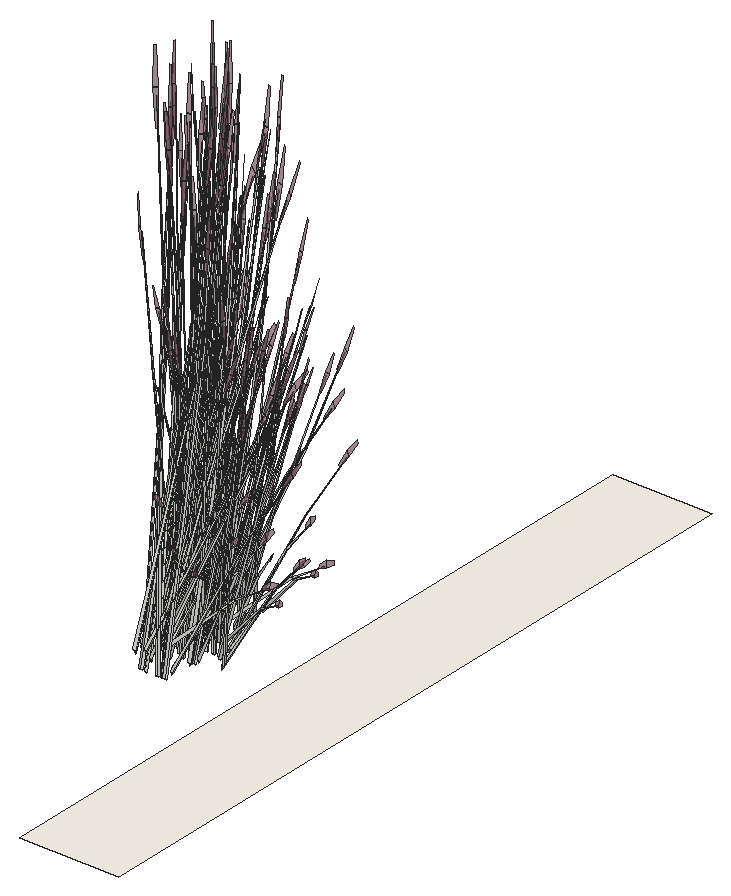
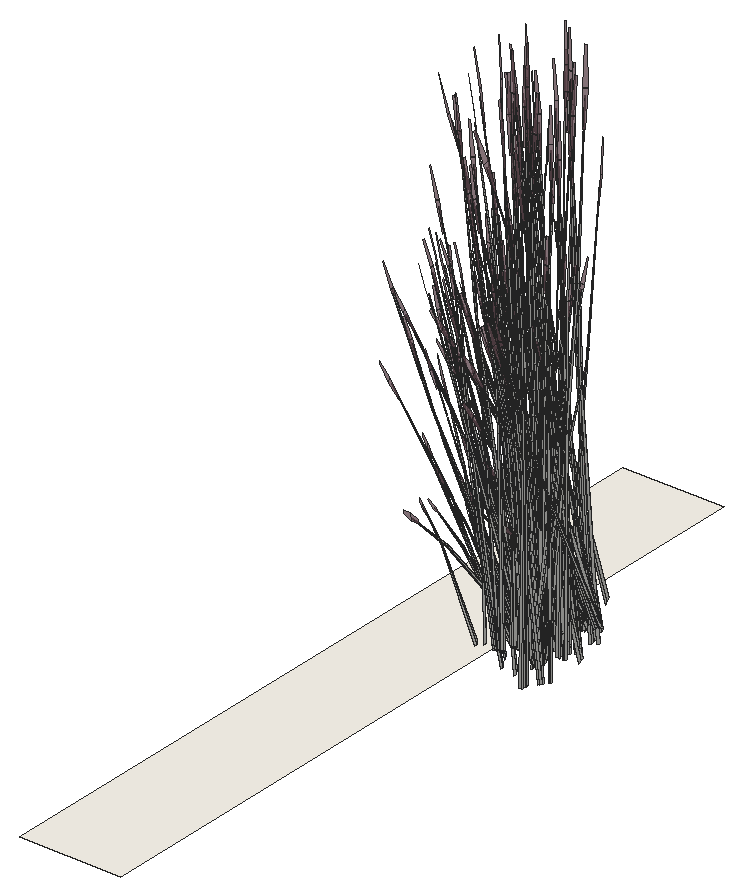
# SketchUp Ruby script. Lengths in inches.
U = 1.inch
M = Sketchup.active_model
def pt(a) = Geom::Point3d.new(a.map { |v| v * U })
def face(e, loops, mat)
  f = e.add_face(loops[0].map { |a| pt(a) })
  loops[1..].each { |l| e.add_face(l.map { |a| pt(a) }).erase! }
  f.material = f.back_material = mat if mat
  f
end
# faces: each face lists its corners as indices into pts; further lists are holes
def faces(e, pts, list, mat = nil) = list.each { |f| face(e, (f[0].is_a?(Array) ? f : [f]).map { |l| l.map { |i| pts[i] } }, mat) }
# xy, xz, yz: faces in a plane at the given z, y or x. An outline is a flat list of corners, or four numbers for a rectangle; further outlines are holes
def ring(l) = l.size == 4 ? [[l[0], l[1]], [l[2], l[1]], [l[2], l[3]], [l[0], l[3]]] : l.each_slice(2).to_a
def flat(e, list, mat, &to3) = list.each { |f| face(e, (f[0].is_a?(Array) ? f : [f]).map { |l| ring(l).map { |u, v| to3.(u, v) } }, mat) }
def xy(e, z, list, mat = nil) = flat(e, list, mat) { |x, y| [x, y, z] }
def xz(e, y, list, mat = nil) = flat(e, list, mat) { |x, z| [x, y, z] }
def yz(e, x, list, mat = nil) = flat(e, list, mat) { |y, z| [x, y, z] }
def lines(e, pts, list) = list.each { |a, b| e.add_line(pt(pts[a]), pt(pts[b])) }
# prism: a flat outline (further loops are holes) pulled along v
def prism(e, loops, v, mat = nil)
  f = face(e, loops, mat); d = Geom::Vector3d.new(v.map { |x| x * U })
  f.pushpull(f.normal.samedirection?(d) ? d.length : -d.length)
end
def box(e, o, s, mat = nil) = prism(e, [[o, [o[0] + s[0], o[1], o[2]], [o[0] + s[0], o[1] + s[1], o[2]], [o[0], o[1] + s[1], o[2]]]], [0, 0, s[2]], mat)
def at(x, y, z, deg = 0) = Geom::Transformation.translation(pt([x, y, z])) * Geom::Transformation.rotation(ORIGIN, Z_AXIS, deg.degrees)
def axes(o, x, y, z) = Geom::Transformation.new([*x, 0, *y, 0, *z, 0, *pt(o).to_a, 1])
def part(name) = M.definitions.add(name)
# library, detail: a bought-in or finely detailed component or shape, given as its bounding box
def library(name, o, s) = part(name).tap { |d| box(d.entities, o, s) }
def detail(e, o, s) = box(e.add_group.entities, o, s)
def put(e, d, t, mat = nil) = e.add_instance(d, t).tap { |i| i.material = mat if mat }
def group(e, t, mat = nil) = e.add_group.tap { |g| g.transformation = t; g.material = mat if mat }.entities
root = M.entities
M.materials.add("C01_Vanilla_Cream").color = [255, 251, 241]
M.materials.add("LightPink_Translucent").color = [144, 107, 117]
M.materials["LightPink_Translucent"].alpha = 0.75
c1 = part("blade")
p = [[2.15,0.21,22],[0,0.17,0],[0.09,0.45,0],[2.18,0.31,22],[2.29,0.31,22],[0.38,0.45,0],
  [2.48,0.24,33],[2.49,0.24,33],[2.48,0.22,33]]
faces(c1.entities,p,[[0,1,2,3],[4,5,2,3],[6,3,4,7],[8,0,3,6]])
c2 = part("seeds")
p = [[0.3,-0.1,1.38],[-0.01,-0.03,1.59],[-0.01,-0.03,0.03],[0.14,-0.07,-0.07],[0.29,-0.03,3],[0.15,0.01,3.11]]
faces(c2.entities,p,[[0,1,2,3],[1,0,4,5]],"LightPink_Translucent")
c3 = part("blade with seeds")
put(c3.entities,c1,at(0,0,0))
put(c3.entities,c2,axes([2.4,0.25,30.99],[1.5799,-0.05474,1.17369],[-0.12525,1.92788,0.29478],[-0.07173,-0.02425,1.56792]))
xy(root,390,[[696.41,288,706,360]],"C01_Vanilla_Cream")
put(root,c3,axes([690.39,317.23,392.17],[0.48065,0.34305,0.12018],[-0.40092,0.38703,-0.34318],[-0.1116,0.05232,1.05198]))
put(root,c3,axes([690.22,316.8125,391.91],[-0.60515,-0.49144,-0.05089],[0.60552,-0.49174,0],[-0.02113,-0.01716,1.45724]))
put(root,c3,axes([690.38,316.98,392.26],[0.70648,-0.03525,0.37133],[0.06389,0.58508,-0.17871],[-0.12647,0.0593,1.19224]))
put(root,c3,axes([687.82,313.22,394.19],[0.19614,-0.43908,0.29394],[0.57222,0.12807,-0.37948],[0.05247,0.17678,0.72609]))
put(root,c3,axes([688.87,312.48,391.9],[0.28286,0.65594,-0.0499],[-0.80821,0.22985,0],[0.00988,0.02291,1.42904]))
put(root,c3,axes([689.42,319.33,393.93],[0.47939,-0.19405,0.05337],[0.23464,0.35385,0.42015],[-0.0463,-0.15598,0.64067]))
put(root,c3,axes([690.9,318.29,392.06],[0.60889,-0.28548,0.4121],[0.36394,0.51192,0],[-0.13868,0.06502,1.30728]))
put(root,c3,axes([689,316.25,391.96],[0.28286,0.63846,0.37976],[-0.80821,0.22202,0.14902],[0.00988,-0.11732,1.31851]))
put(root,c3,axes([689.25,319.36,393.93],[0.64106,0.14927,0.39842],[-0.21921,0.49074,0.32852],[-0.03852,-0.19299,0.82444]))
put(root,c3,axes([688.87,316.16,391.83],[0.31565,-0.51449,-0.37133],[0.65588,0.24761,0.17871],[0,-0.1186,1.19224]))
put(root,c3,axes([688.48,321.81,392.02],[0.73304,0.27674,0.19974],[-0.35279,0.57501,0.41502],[0,-0.13255,1.3325]))
put(root,c3,axes([689.68,317.82,391.83],[-0.21227,-0.49226,0],[0.60616,-0.17239,0],[0,0,1.28128]))
put(root,c3,axes([687.9375,313.28,394.13],[0.31051,0.46426,-0.58968],[-0.63919,0.25873,0.07116],[0.07261,0.22432,0.83415]))
put(root,c3,axes([691.21,311.62,391.83],[-0.81312,-0.00457,-0.0413],[0,-0.63814,0.41452],[-0.02555,0.14527,1.31432]))
put(root,c3,axes([688.59,314.78,394.6875],[0.44958,-0.32756,-0.05385],[0.41194,0.35875,-0.24415],[0.029,0.10165,0.8053]))
put(root,c3,axes([687.58,319.72,391.97],[-0.40676,-0.57214,0],[0.68052,-0.31907,-0.42834],[0.15499,-0.07267,1.3588]))
put(root,c3,axes([690.54,316.85,391.83],[-0.31565,0.51449,-0.37133],[-0.65588,-0.24761,0.17871],[0,0.1186,1.19224]))
put(root,c3,axes([689.11,312.7,391.83],[0.65588,0.25634,0],[-0.31565,0.53263,0],[0,0,1.45212]))
put(root,c3,axes([688.17,313.38,393.89],[0.63954,0.14313,-0.42412],[-0.21921,0.49074,-0.32852],[0.05864,0.19758,0.81151]))
put(root,c3,axes([687.625,313.4,394.18],[0.63664,-0.26583,-0.10093],[0.31286,0.47181,-0.56021],[0.084,0.19882,0.85122]))
put(root,c3,axes([691.78,316.54,392.05],[-0.51116,-0.4159,0.14643],[0.51512,-0.4034,0.29122],[-0.05645,0.08494,1.33138]))
put(root,c3,axes([690.02,316.3,391.83],[0,-0.66065,0],[0.81352,0,0],[0,0,1.48949]))
put(root,c3,axes([689.28,318.33,392.3],[0.08346,0.33295,0.95334],[-0.46298,-0.1844,0.70045],[0.04982,-0.17048,0.20998]))
put(root,c3,axes([689.26,316.42,392.02],[0.73304,0.27674,0.19974],[-0.35279,0.57501,0.41502],[0,-0.13255,1.3325]))
put(root,c3,axes([690.43,316.5625,391.9],[0,0.66033,-0.04679],[-0.81352,0,0],[0,0.02075,1.48875]))
put(root,c3,axes([689.03,316.03,392.26],[-0.70648,0.03525,0.37133],[-0.06389,-0.58508,-0.17871],[0.12647,-0.0593,1.19224]))
put(root,c3,axes([691.04,311.72,391.68],[-0.45414,0.35624,-0.25712],[-0.45414,-0.35624,0.25712],[0,0.11474,1.15348]))
put(root,c3,axes([689.74,311.65,391.74],[0.23855,0.52277,-0.57446],[-0.68718,0.18827,-0.15077],[0.02637,0.17702,1.26801]))
put(root,c3,axes([688.7,315.03,392.05],[-0.18794,0.56744,0.14643],[-0.68774,-0.16058,0.29122],[0.1188,-0.00276,1.33138]))
put(root,c3,axes([690.04,317.84,391.9],[0.28286,0.65594,-0.0499],[-0.80821,0.22985,0],[0.00988,0.02291,1.42904]))
put(root,c3,axes([691.26,318.88,393.91],[-0.06607,0.04361,1.47228],[-0.64734,-0.14714,-0.13912],[-0.02343,-0.19032,0.26054]))
put(root,c3,axes([690.75,320.14,394.18],[-0.71502,-0.02829,-0.10093],[0.01954,-0.53563,-0.56021],[0.04967,-0.20629,0.85122]))
put(root,c3,axes([692.375,316.98,391.83],[-0.81312,-0.00457,-0.0413],[0,-0.63814,0.41452],[-0.02555,0.14527,1.31432]))
put(root,c3,axes([689.45,311.07,392.21],[0.73268,0.27244,-0.24149],[-0.35279,0.57501,-0.41502],[0.02303,0.14118,1.32557]))
put(root,c3,axes([690.78,315.0625,392.05],[-0.6991,0.15154,0.14643],[-0.17263,-0.56398,0.29122],[0.06235,0.08217,1.33138]))
put(root,c3,axes([690.47,320.22,394.19],[-0.4402,0.30062,0.29394],[-0.41671,-0.34326,-0.37948],[0.0634,-0.1744,0.72609]))
put(root,c3,axes([688.375,321.3,392.21],[-0.07581,-0.65151,-0.24149],[0.7896,-0.03939,-0.41502],[0.13904,-0.08678,1.32557]))
put(root,c3,axes([690.27,319.93,393.89],[-0.46573,-0.38364,-0.42412],[0.49199,-0.33598,-0.32852],[0.07086,-0.19492,0.81151]))
put(root,c3,axes([689.63,315.88,391.96],[-0.53943,0.51816,0.37976],[-0.64086,-0.4574,0.14902],[0.13005,-0.05171,1.31851]))
put(root,c3,axes([690.55,316.7,391.84],[0.45414,0.3688,0],[-0.45414,0.3688,0],[0,0,1.40491]))
put(root,c3,axes([690.55,316.27,392.26],[0.31565,-0.51449,0.37133],[0.65588,0.24761,-0.17871],[0,0.1186,1.19224]))
put(root,c3,axes([690.27,318.06,391.83],[0.65588,0.25634,0],[-0.31565,0.53263,0],[0,0,1.45212]))
put(root,c3,axes([691.35,311.73,391.67],[0,0.57097,-0.4121],[-0.72788,0,0],[0,0.13004,1.30728]))
put(root,c3,axes([689.4,313.46,393.93],[-0.64708,0.13103,0.39842],[-0.1123,-0.514,0.32852],[0.15218,0.15149,0.82444]))
put(root,c3,axes([689.28,313.56,393.93],[-0.29569,0.36271,0.05337],[-0.42107,-0.21117,0.42015],[0.13613,0.11629,0.64067]))
put(root,c3,axes([688.53,312.36,393.22],[-0.14872,-0.18332,1.42242],[0.6872,-0.15433,0.11501],[0.15531,0.28779,0.60807]))
put(root,c3,axes([688.27,319.85,391.68],[0.60696,0.14127,-0.25712],[-0.15283,0.49751,0.25712],[0.12236,-0.05737,1.15348]))
put(root,c3,axes([690.34,316.15,391.98],[-0.82229,-0.1203,0.40835],[0.16734,-0.67942,0.16024],[0.12017,0.06561,1.41775]))
put(root,c3,axes([689.96,319.25,392.15],[-0.18493,0.11557,1.18691],[-0.55384,-0.20228,-0.25526],[0.10266,-0.25157,0.50747]))
put(root,c3,axes([692.21,317.07,391.68],[-0.45414,0.35624,-0.25712],[-0.45414,-0.35624,0.25712],[0,0.11474,1.15348]))
put(root,c3,axes([688.13,319.63,391.67],[0.60889,-0.28548,-0.4121],[0.36394,0.51192,0],[0.13868,-0.06502,1.30728]))
put(root,c3,axes([690.57,316.45,391.83],[0.72788,0,0],[0,0.59111,0],[0,0,1.48078]))
put(root,c3,axes([689.87,315.8,392.26],[-0.39083,-0.47924,0.37133],[0.59199,-0.33747,-0.17871],[0.12647,0.0593,1.19224]))
put(root,c3,axes([689.16,315.91,392.21],[-0.07581,-0.65151,-0.24149],[0.7896,-0.03939,-0.41502],[0.13904,-0.08678,1.32557]))
put(root,c3,axes([690.82,316.39,392.17],[0.60616,-0.16651,0.12018],[0.21227,0.47548,-0.34318],[0,0.10465,1.05198]))
put(root,c3,axes([690.41,320.11,394.13],[0.01693,-0.52814,-0.58968],[0.71285,0.03547,0.07116],[0.07523,-0.22375,0.83415]))
put(root,c3,axes([689.1875,313.14,394.19],[-0.10048,-0.4599,0.29394],[0.5744,-0.12144,-0.37948],[0.15428,0.13179,0.72609]))
put(root,c3,axes([690.62,316.43,392.21],[0.73268,0.27244,-0.24149],[-0.35279,0.57501,-0.41502],[0.02303,0.14118,1.32557]))
put(root,c3,axes([689.06,314.47,391.68],[0.60696,0.14127,-0.25712],[-0.15283,0.49751,0.25712],[0.12236,-0.05737,1.15348]))
put(root,c3,axes([689.58,310.5,393.71],[-0.56218,-0.29666,1.14775],[0.59361,-0.46189,0.49522],[0.18138,0.27836,1.10941]))
put(root,c3,axes([688.63,313.79,393.91],[0.00193,-0.06913,1.47228],[0.55753,-0.30498,-0.13912],[0.19366,0.10886,0.26054]))
put(root,c3,axes([690.42,312.91,392.3],[-0.36631,-0.16417,0.95334],[0.47299,-0.16681,0.70045],[0.12758,0.1413,0.20998]))
put(root,c3,axes([689.12,312.74,392.15],[0.01148,-0.18927,1.18691],[0.54864,-0.21141,-0.25526],[0.16937,0.22654,0.50747]))
put(root,c3,axes([692.21,316.56,392.06],[0,-0.57097,0.4121],[0.72788,0,0],[0,0.13004,1.30728]))
put(root,c3,axes([690.13,315.66,392.17],[0.12551,-0.50956,0.12018],[0.6132,0.08845,-0.34318],[0.1116,0.05232,1.05198]))
put(root,c3,axes([690.7,319.79,393.76],[0.4402,-0.30062,-0.29394],[0.41671,0.34326,0.37948],[0.0634,-0.1744,0.72609]))
put(root,c3,axes([690.87,319.95,393.93],[0.53464,0.0266,0.05337],[-0.01466,0.40172,0.42015],[0.05594,-0.15388,0.64067]))
put(root,c3,axes([691.53,311.29,391.97],[0.81352,0,0],[0,0.63814,-0.42834],[0,0.14534,1.3588]))
put(root,c3,axes([691.01,314.77,392.06],[-0.60889,-0.28548,0.4121],[0.36394,-0.51192,0],[0.13868,0.06502,1.30728]))
put(root,c3,axes([691.4,319.29,393.91],[-0.00628,-0.11364,1.45204],[-0.53042,-0.32843,-0.22964],[0.08201,-0.19909,0.11645]))
put(root,c3,axes([688.85,320.8,391.71],[0.43821,-0.42916,-0.51753],[0.54436,0.38915,-0.13583],[0.1756,-0.10706,1.14236]))
put(root,c3,axes([690.7,319.91,393.93],[0.46327,0.38957,0.39842],[-0.49199,0.33598,0.32852],[0.08546,-0.18277,0.82444]))
put(root,c3,axes([690.47,317.75,391.8125],[0.68303,-0.19373,-0.15934],[0.24001,0.55805,0.00007],[0.07539,-0.02141,1.44335]))
put(root,c3,axes([690.48,313.66,392.21],[-0.4172,-0.01791,0.872],[0.27552,-0.38032,0.48145],[0.16481,0.13512,0.68401]))
put(root,c3,axes([690.49,316.1,391.83],[0.39083,0.47924,-0.37133],[-0.59199,0.33747,0.17871],[0.12647,0.0593,1.19224]))
put(root,c3,axes([691.24,321.15,394.19],[-0.56631,0.0816,0.29394],[-0.14954,-0.46647,-0.37948],[0.16229,-0.12529,0.72609]))
put(root,c3,axes([689.14,313.38,394.18],[0.38768,-0.48872,-0.10093],[0.56143,0.28156,-0.56021],[0.19516,0.13808,0.85122]))
put(root,c3,axes([689.61,319.84,393.22],[-0.12114,0.19625,1.42242],[-0.50818,-0.40613,0.11501],[0.22925,-0.25313,0.60807]))
put(root,c3,axes([689.63,315.41,391.71],[0.43821,-0.42916,-0.51753],[0.54436,0.38915,-0.13583],[0.1756,-0.10706,1.14236]))
put(root,c3,axes([689.6,313.14,393.89],[0.64198,-0.13573,-0.42412],[0.1123,0.514,-0.32852],[0.17243,0.1473,0.81151]))
put(root,c3,axes([690.33,312.52,394.19],[-0.37017,-0.35748,0.29394],[0.42268,-0.3384,-0.37948],[0.21476,0.05149,0.72609]))
put(root,c3,axes([691.53,321.19,394.18],[-0.60181,-0.31483,-0.10093],[0.34671,-0.45593,-0.56021],[0.17003,-0.15849,0.85122]))
put(root,c3,axes([691.56,315.03,391.68],[0.15283,0.49751,-0.25712],[-0.60696,0.14127,0.25712],[0.12236,0.05737,1.15348]))
put(root,c3,axes([692.7,316.65,391.97],[0.81352,0,0],[0,0.63814,-0.42834],[0,0.14534,1.3588]))
put(root,c3,axes([690.67,312.85,393.93],[-0.03276,0.43418,0.05337],[-0.49468,-0.0119,0.42015],[0.18949,0.04543,0.64067]))
put(root,c3,axes([690.53,313.52,391.24],[0.0474,-0.08243,1.46364],[0.59674,-0.24277,-0.2236],[0.18092,0.12565,0.24931]))
put(root,c3,axes([690.71,312.71,393.93],[-0.47971,0.37622,0.39842],[-0.41372,-0.39954,0.32852],[0.22506,0.0694,0.82444]))
put(root,c3,axes([690.07,315.83,392.21],[0.65687,-0.37907,-0.24149],[0.43681,0.53562,-0.41502],[0.16207,0.0544,1.32557]))
put(root,c3,axes([692.02,315.76,394.19],[-0.56631,0.0816,0.29394],[-0.14954,-0.46647,-0.37948],[0.16229,-0.12529,0.72609]))
put(root,c3,axes([691.25,319.61,391.24],[-0.09738,-0.04498,1.46364],[-0.25012,-0.50252,-0.2236],[0.16873,-0.13637,0.24931]))
put(root,c3,axes([691.23,320.82,393.89],[-0.16713,-0.52135,-0.42412],[0.63294,-0.0912,-0.32852],[0.18138,-0.14003,0.81151]))
put(root,c3,axes([688.41,315.49,391.32],[-0.64037,0.22859,1.07011],[-0.20382,-0.65589,0.4158],[0.39323,0.01091,1.21713]))
put(root,c3,axes([691.36,314.47,391.97],[0.40676,-0.57214,0],[0.68052,0.31907,-0.42834],[0.15499,0.07267,1.3588]))
put(root,c3,axes([692.01,319.78,392.3],[-0.2167,0.29065,0.95334],[-0.18626,-0.3905,0.70045],[0.17898,-0.09785,0.20998]))
put(root,c3,axes([689.53,311.79,393.22],[-0.24166,-0.09837,1.42242],[0.50011,-0.41269,0.11501],[0.3117,0.18617,0.60807]))
put(root,c3,axes([691.75,321.07,393.93],[0.44663,0.24013,0.05337],[-0.26003,0.34195,0.42015],[0.14319,-0.11055,0.64067]))
put(root,c3,axes([691.5,317.88,394.19],[-0.37017,-0.35748,0.29394],[0.42268,-0.3384,-0.37948],[0.21476,0.05149,0.72609]))
put(root,c3,axes([691.73,314.82,391.67],[0.60889,0.28548,-0.4121],[-0.36394,0.51192,0],[0.13868,0.06502,1.30728]))
put(root,c3,axes([691.625,320.97,393.93],[0.16135,0.52549,0.39842],[-0.63294,0.0912,0.32852],[0.18654,-0.12359,0.82444]))
put(root,c3,axes([691.84,318.2,393.93],[-0.03276,0.43418,0.05337],[-0.49468,-0.0119,0.42015],[0.18949,0.04543,0.64067]))
put(root,c3,axes([691.88,318.07,393.93],[-0.47971,0.37622,0.39842],[-0.41372,-0.39954,0.32852],[0.22506,0.0694,0.82444]))
put(root,c3,axes([690.86,312.71,393.76],[0.37017,0.35748,-0.29394],[-0.42268,0.3384,0.37948],[0.21476,0.05149,0.72609]))
put(root,c3,axes([693.13,318.12,393.26],[-0.12452,-0.47997,-0.02898],[0.58854,-0.11034,-0.1314],[0.1229,0.03043,0.43341]))
put(root,c3,axes([692.11,316.88,394.19],[-0.54068,-0.15928,0.29394],[0.1577,-0.46469,-0.37948],[0.21769,-0.04261,0.72609]))
put(root,c3,axes([693.01,321.05,393.91],[-0.08498,-0.00434,1.47228],[-0.35287,-0.46464,-0.13912],[0.14171,-0.15278,0.26054]))
put(root,c3,axes([690.84,315.91,391.71],[0.67676,0.09361,-0.51753],[-0.14281,0.57742,-0.13583],[0.20196,0.06997,1.14236]))
put(root,c3,axes([691.7,320.87,393.76],[0.56631,-0.0816,-0.29394],[0.14954,0.46647,0.37948],[0.16229,-0.12529,0.72609]))
put(root,c3,axes([693.72,316.25,391.875],[-0.40335,-0.3651,-0.05385],[0.44175,-0.33453,-0.24415],[0.12517,-0.02355,0.8053]))
put(root,c3,axes([691.25,321.03,394.13],[0.33983,-0.45051,-0.58968],[0.59551,0.32017,0.07116],[0.20291,-0.16322,0.83415]))
put(root,c3,axes([692.79,314.39,392.3],[-0.2167,0.29065,0.95334],[-0.18626,-0.3905,0.70045],[0.17898,-0.09785,0.20998]))
put(root,c3,axes([692.54,315.6875,393.93],[0.44663,0.24013,0.05337],[-0.26003,0.34195,0.42015],[0.14319,-0.11055,0.64067]))
put(root,c3,axes([691.01,312.4,393.91],[0.13956,-0.00966,1.45204],[0.38281,-0.44358,-0.22964],[0.24825,0.05855,0.11645]))
put(root,c3,axes([692.41,315.59,393.93],[0.16135,0.52549,0.39842],[-0.63294,0.0912,0.32852],[0.18654,-0.12359,0.82444]))
put(root,c3,axes([693.8,315.67,393.91],[-0.08498,-0.00434,1.47228],[-0.35287,-0.46464,-0.13912],[0.14171,-0.15278,0.26054]))
put(root,c3,axes([692.48,315.49,393.76],[0.56631,-0.0816,-0.29394],[0.14954,0.46647,0.37948],[0.16229,-0.12529,0.72609]))
put(root,c3,axes([692.6,317.02,393.93],[0.23895,0.38931,0.05337],[-0.43573,0.19055,0.42015],[0.19208,-0.0376,0.64067]))
put(root,c3,axes([692.03,318.07,393.76],[0.37017,0.35748,-0.29394],[-0.42268,0.3384,0.37948],[0.21476,0.05149,0.72609]))
put(root,c3,axes([690.47,312.47,394.13],[0.65035,0.01375,-0.58968],[-0.04368,0.5789,0.07116],[0.27552,0.06109,0.83415]))
put(root,c3,axes([691.6,318.11,394.18],[0.03484,-0.58066,-0.10093],[0.65957,0.01587,-0.56021],[0.25402,0.04034,0.85122]))
put(root,c3,axes([692.34,317.03,394.18],[-0.32734,-0.51701,-0.10093],[0.58097,-0.25407,-0.56021],[0.24483,-0.06821,0.85122]))
put(root,c3,axes([692.56,316.88,393.93],[-0.18381,0.5206,0.39842],[-0.60429,-0.17802,0.32852],[0.23764,-0.03129,0.82444]))
put(root,c3,axes([691.74,320.61,392.15],[-0.23242,-0.01691,1.18691],[-0.23811,-0.45367,-0.25526],[0.28553,-0.12834,0.50747]))
put(root,c3,axes([692.18,317.76,393.91],[0.13956,-0.00966,1.45204],[0.38281,-0.44358,-0.22964],[0.24825,0.05855,0.11645]))
put(root,c3,axes([692.3125,316.59,393.89],[0.17625,-0.51936,-0.42412],[0.60429,0.17802,-0.32852],[0.2433,-0.04762,0.81151]))
put(root,c3,axes([693.83,316.92,392.3],[-0.40197,0.09426,0.95334],[0.18921,-0.38956,0.70045],[0.21325,0.02666,0.20998]))
put(root,c3,axes([692.68,316.83,393.76],[0.54068,0.15928,-0.29394],[-0.1577,0.46469,0.37948],[0.21769,-0.04261,0.72609]))
put(root,c3,axes([691.91,312.1875,392.15],[-0.15668,-0.14043,1.18691],[0.20386,-0.46454,-0.25526],[0.31701,0.06293,0.50747]))
put(root,c3,axes([693.33,321.61,393.91],[0.09028,-0.08697,1.45204],[-0.11555,-0.53348,-0.22964],[0.22652,-0.10115,0.11645]))
put(root,c3,axes([691.64,317.83,394.13],[0.65035,0.01375,-0.58968],[-0.04368,0.5789,0.07116],[0.27552,0.06109,0.83415]))
put(root,c3,axes([692.96,316.74,391.65],[-0.41902,0.06852,1.17514],[-0.0667,-0.54541,0.06726],[0.29348,-0.08255,0.6687]))
put(root,c3,axes([693.41,316.38,391.24],[-0.034,-0.08668,1.46364],[0.23582,-0.50706,-0.2236],[0.23788,-0.00729,0.24931]))
put(root,c3,axes([693.64,318.57,393.91],[-0.05883,-0.04999,1.47228],[0.12868,-0.53581,-0.13912],[0.23172,-0.03423,0.26054]))
put(root,c3,axes([691.21,316.25,393.22],[-0.26985,0.01293,1.42242],[0.17902,-0.56047,0.11501],[0.38456,0.03467,0.60807]))
put(root,c3,axes([692.2,316.78,394.13],[0.57168,-0.25217,-0.58968],[0.3186,0.51908,0.07116],[0.27622,-0.05897,0.83415]))
put(root,c3,axes([694.12,316.22,393.91],[0.09028,-0.08697,1.45204],[-0.11555,-0.53348,-0.22964],[0.22652,-0.10115,0.11645]))
put(root,c3,axes([693.08,317.55,392.15],[-0.15668,-0.14043,1.18691],[0.20386,-0.46454,-0.25526],[0.31701,0.06293,0.50747]))
